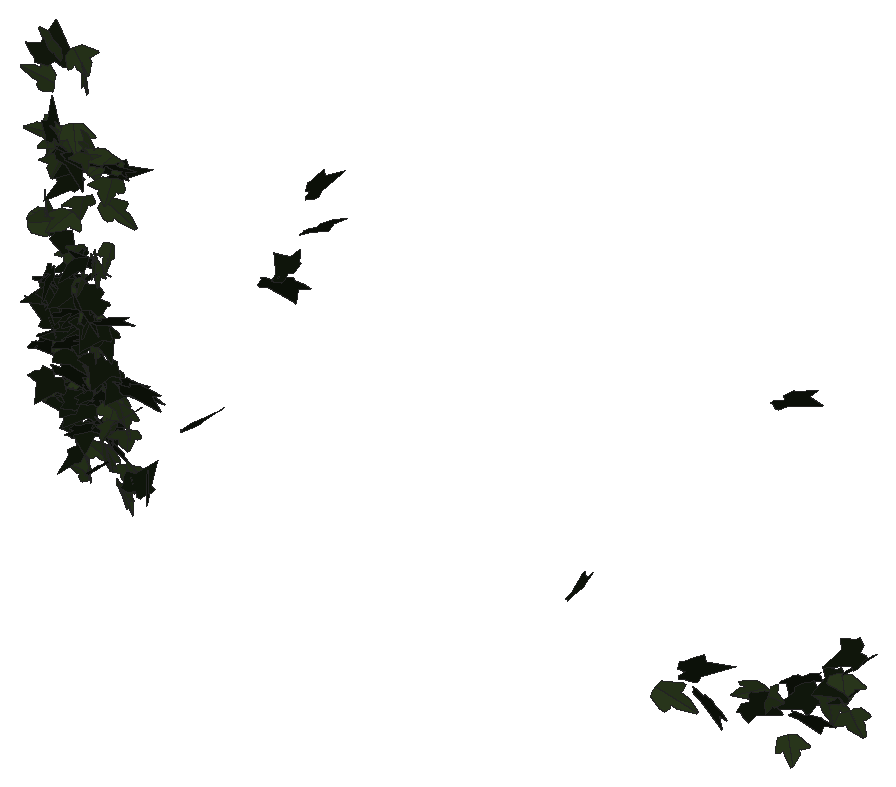
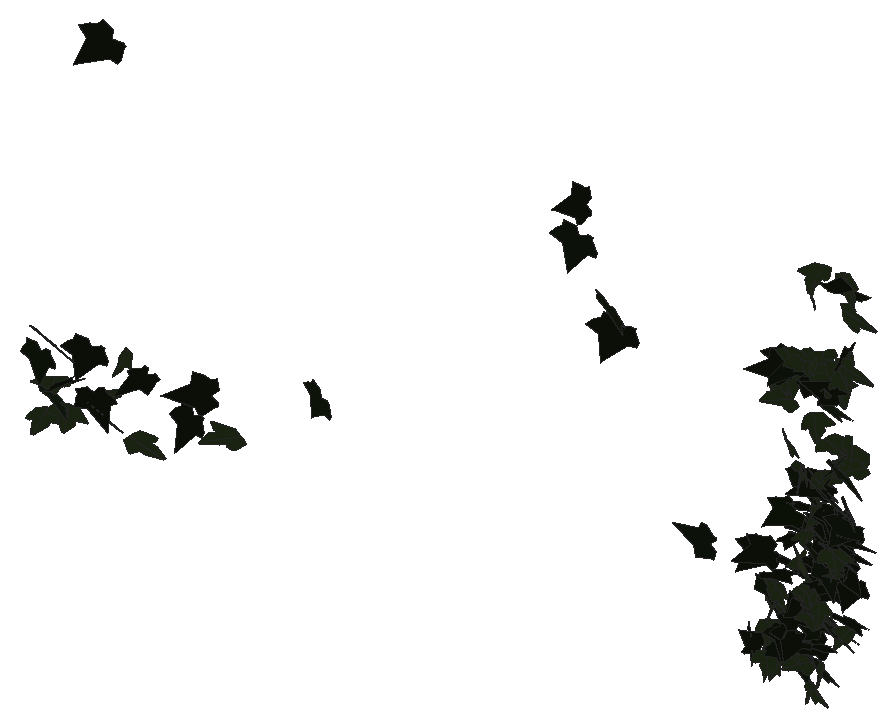
# SketchUp Ruby script. Lengths in inches.
U = 1.inch
M = Sketchup.active_model
def pt(a) = Geom::Point3d.new(a.map { |v| v * U })
def face(e, loops, mat)
  f = e.add_face(loops[0].map { |a| pt(a) })
  loops[1..].each { |l| e.add_face(l.map { |a| pt(a) }).erase! }
  f.material = f.back_material = mat if mat
  f
end
# faces: each face lists its corners as indices into pts; further lists are holes
def faces(e, pts, list, mat = nil) = list.each { |f| face(e, (f[0].is_a?(Array) ? f : [f]).map { |l| l.map { |i| pts[i] } }, mat) }
# xy, xz, yz: faces in a plane at the given z, y or x. An outline is a flat list of corners, or four numbers for a rectangle; further outlines are holes
def ring(l) = l.size == 4 ? [[l[0], l[1]], [l[2], l[1]], [l[2], l[3]], [l[0], l[3]]] : l.each_slice(2).to_a
def flat(e, list, mat, &to3) = list.each { |f| face(e, (f[0].is_a?(Array) ? f : [f]).map { |l| ring(l).map { |u, v| to3.(u, v) } }, mat) }
def xy(e, z, list, mat = nil) = flat(e, list, mat) { |x, y| [x, y, z] }
def xz(e, y, list, mat = nil) = flat(e, list, mat) { |x, z| [x, y, z] }
def yz(e, x, list, mat = nil) = flat(e, list, mat) { |y, z| [x, y, z] }
def lines(e, pts, list) = list.each { |a, b| e.add_line(pt(pts[a]), pt(pts[b])) }
# prism: a flat outline (further loops are holes) pulled along v
def prism(e, loops, v, mat = nil)
  f = face(e, loops, mat); d = Geom::Vector3d.new(v.map { |x| x * U })
  f.pushpull(f.normal.samedirection?(d) ? d.length : -d.length)
end
def box(e, o, s, mat = nil) = prism(e, [[o, [o[0] + s[0], o[1], o[2]], [o[0] + s[0], o[1] + s[1], o[2]], [o[0], o[1] + s[1], o[2]]]], [0, 0, s[2]], mat)
def at(x, y, z, deg = 0) = Geom::Transformation.translation(pt([x, y, z])) * Geom::Transformation.rotation(ORIGIN, Z_AXIS, deg.degrees)
def axes(o, x, y, z) = Geom::Transformation.new([*x, 0, *y, 0, *z, 0, *pt(o).to_a, 1])
def part(name) = M.definitions.add(name)
# library, detail: a bought-in or finely detailed component or shape, given as its bounding box
def library(name, o, s) = part(name).tap { |d| box(d.entities, o, s) }
def detail(e, o, s) = box(e.add_group.entities, o, s)
def put(e, d, t, mat = nil) = e.add_instance(d, t).tap { |i| i.material = mat if mat }
def group(e, t, mat = nil) = e.add_group.tap { |g| g.transformation = t; g.material = mat if mat }.entities
root = M.entities
M.materials.add("1026 AP 7946 SUNNY SIDE UP").color = [254, 231, 186]
M.materials.add("efeu1").color = [18, 25, 13]
M.materials.add("efeu2").color = [43, 57, 29]
c1 = part("ivyleaf_10")
p = [[0,0.5,-0.03],[-0.0625,2.02,-0.43],[-0.19,2.01,-0.46],[-0.54,1.05,-0.29],[-0.52,0.625,-0.18],[-0.83,0.76,-0.28],
  [-1.16,0.64,-0.33],[-1.15,0.33,-0.24],[-0.77,-0.39,0.02],[-0.3,-0.51,0.16],[0.04,-0.48,0.23],[-0.02,2.01,-0.4375],
  [-0.06,2.01,-0.43],[0.04,-0.49,0.23],[0.67,-0.49,0.14],[1.38,0.36,-0.2],[1.375,0.51,-0.24],[0.81,0.65,-0.19],
  [0.62,0.59,-0.15],[0.6,1.09,-0.28],[0.5,1.23,-0.31]]
faces(c1.entities,p,[[0,1,2,3,4,5,6,7,8,9,10],[11,12,0,13,14,15,16,17,18,19,20]],"efeu2")
c2 = part("ivyleaf_9")
p = [[1.54,2.16,1.25],[1.36,2.04,1.19],[-0.21,0.99,0.68],[-0.71,1.11,0.82],[-0.85,0.86,0.67],[-0.8,0.17,0.21],
  [-0.9,-0.01,0.1],[-0.67,-0.16,-0.02],[-0.08,-0.08,-0.05],[-0.03,-0.6,-0.4],[0.65,-0.88,-0.66],[0.83,-0.6,-0.49],
  [1.29,-0.42,-0.43],[1.8125,-0.07,-0.26],[1.21,0.44,0.15]]
faces(c2.entities,p,[[0,1,2,3,4,5,6,7,8,9,10,11,12,13,14]],"efeu1")
put(root,c1,axes([98.42,213.14,277.24],[0.01091,0.05162,0.27942],[-0.44913,0.02167,0.0027],[-0.03534,-0.2595,0.05202]),"1026 AP 7946 SUNNY SIDE UP")
put(root,c1,axes([98.55,213.2,275.9],[-0.07101,0.03292,0.2675],[-0.42315,-0.03971,-0.0397],[0.05791,-0.24978,0.03794]),"1026 AP 7946 SUNNY SIDE UP")
put(root,c1,axes([98.3125,213.24,274.14],[-0.23454,0.18097,0.09974],[-0.13964,0.05028,-0.24058],[-0.31407,-0.1575,0.03248]),"1026 AP 7946 SUNNY SIDE UP")
put(root,c1,axes([98.02,213.31,273.63],[0.17305,0.09582,0.20323],[0.2394,0.12524,-0.14799],[-0.26763,0.17399,-0.00097]),"1026 AP 7946 SUNNY SIDE UP")
put(root,c1,axes([98.4375,213.24,278.14],[-0.33536,0.12077,0.14156],[-0.23164,0.02245,-0.24278],[-0.19382,-0.23579,0.04521]),"1026 AP 7946 SUNNY SIDE UP")
put(root,c2,axes([98.49,213.48,271.78],[-0.34588,-0.02797,0.10109],[-0.14748,-0.05284,-0.21736],[0.07996,-0.21842,0.03636]),"1026 AP 7946 SUNNY SIDE UP")
put(root,c2,axes([98.21,213.35,272.16],[0.28691,0.14385,0.05154],[0.01081,0.06257,-0.23231],[-0.25628,0.16368,0.0479]),"1026 AP 7946 SUNNY SIDE UP")
put(root,c2,axes([98.27,213.1875,270.64],[0.2103,0.18763,-0.0042],[0.01051,-0.01171,-0.24055],[-0.31852,0.12349,-0.01071]),"1026 AP 7946 SUNNY SIDE UP")
put(root,c2,axes([98.5,213.48,273.58],[-0.24446,0.18597,-0.01038],[-0.00582,-0.01796,-0.25164],[-0.31631,-0.1434,0.01265]),"1026 AP 7946 SUNNY SIDE UP")
put(root,c1,axes([98.17,213.02,273.62],[-0.00352,-0.01577,0.26143],[0.1187,0.23419,0.02008],[-0.39843,0.06991,0.00367]),"1026 AP 7946 SUNNY SIDE UP")
put(root,c2,axes([98.65,213.15,271.35],[-0.11475,0.11007,0.21516],[-0.25252,0.13636,-0.13257],[-0.29305,-0.1606,0.02999]),"1026 AP 7946 SUNNY SIDE UP")
put(root,c2,axes([98.44,213.28,269.74],[-0.33804,-0.05996,-0.05433],[0.09397,-0.01196,-0.22097],[0.09341,-0.20496,0.02568]),"1026 AP 7946 SUNNY SIDE UP")
put(root,c1,axes([98.34,213.3,269.43],[0.08571,0.15443,0.15045],[-0.00221,0.14279,-0.16793],[-0.35215,0.03669,0.03767]),"1026 AP 7946 SUNNY SIDE UP")
put(root,c2,axes([98.4375,213.1,271.4],[0.20472,-0.0542,-0.20479],[-0.29694,0.07567,-0.14048],[0.15798,0.21246,0.00133]),"1026 AP 7946 SUNNY SIDE UP")
put(root,c1,axes([98.49,213.35,275.81],[0.03464,0.23008,-0.09791],[-0.14517,-0.0825,-0.23609],[-0.39646,0.05031,0.07789]),"1026 AP 7946 SUNNY SIDE UP")
put(root,c2,axes([98.6,213.23,270.97],[-0.01316,0.1754,-0.14964],[-0.05252,-0.14163,-0.18737],[-0.37954,0.01352,0.03112]),"1026 AP 7946 SUNNY SIDE UP")
put(root,c2,axes([98.55,213.21,277.77],[-0.42037,0.02729,0.08947],[0.14494,0.01969,0.26537],[0.03308,0.2605,-0.02574]),"1026 AP 7946 SUNNY SIDE UP")
put(root,c2,axes([98.42,213.22,272.4375],[-0.20286,0.03865,-0.21315],[0.29531,-0.10039,-0.13371],[-0.17862,-0.20987,0.02101]),"1026 AP 7946 SUNNY SIDE UP")
put(root,c1,axes([98.61,213.22,275.73],[-0.21138,-0.17852,-0.14178],[-0.15191,-0.09578,0.23105],[-0.34284,0.15251,-0.01497]),"1026 AP 7946 SUNNY SIDE UP")
put(root,c2,axes([98.51,213.375,272.24],[0.27432,0.15021,-0.04954],[-0.03663,-0.04736,-0.23593],[-0.26529,0.16186,-0.01865]),"1026 AP 7946 SUNNY SIDE UP")
put(root,c2,axes([98.48,213.49,271.73],[-0.18652,-0.19675,0.02288],[0.06417,-0.04767,-0.23437],[0.33028,-0.10185,0.05846]),"1026 AP 7946 SUNNY SIDE UP")
put(root,c1,axes([98.6,213.47,271.35],[-0.2889,-0.1418,0.03043],[-0.00796,-0.04127,-0.23577],[0.24601,-0.16786,0.02811]),"1026 AP 7946 SUNNY SIDE UP")
put(root,c2,axes([98.72,213.48,269.5625],[-0.27699,0.12648,-0.04289],[0.03306,-0.04259,-0.22043],[-0.22364,-0.16294,0.02053]),"1026 AP 7946 SUNNY SIDE UP")
put(root,c2,axes([98.58,213.34,272.32],[0.17219,0.19894,-0.03572],[-0.01358,-0.03625,-0.23937],[-0.34291,0.10133,-0.00846]),"1026 AP 7946 SUNNY SIDE UP")
put(root,c2,axes([98.63,213.08,275.96],[-0.12376,-0.12351,0.23299],[0.1538,0.20006,0.15571],[-0.39851,0.11557,-0.01226]),"1026 AP 7946 SUNNY SIDE UP")
put(root,c1,axes([98.59,213.48,270.85],[0.18494,0.14833,-0.13167],[-0.10181,-0.11049,-0.198],[-0.31307,0.12356,-0.0134]),"1026 AP 7946 SUNNY SIDE UP")
put(root,c2,axes([98.9,213.25,271.31],[-0.15454,0.17398,0.12199],[-0.18019,0.06538,-0.20077],[-0.30117,-0.12839,0.05752]),"1026 AP 7946 SUNNY SIDE UP")
put(root,c2,axes([98.75,213.51,270.94],[-0.00684,0.22013,-0.00663],[0.00213,-0.00904,-0.23582],[-0.37398,-0.00408,-0.00122]),"1026 AP 7946 SUNNY SIDE UP")
put(root,c1,axes([98.75,213.17,275.4],[-0.18203,-0.22494,0.06303],[-0.02963,-0.0601,-0.26742],[0.39489,-0.1082,0.00899]),"1026 AP 7946 SUNNY SIDE UP")
put(root,c2,axes([98.82,213.28,273.22],[-0.13782,-0.18844,0.13747],[0.0698,0.12462,0.22116],[-0.38315,0.09049,-0.00916]),"1026 AP 7946 SUNNY SIDE UP")
put(root,c1,axes([98.88,213.23,273.96],[0.2441,0.12071,-0.15989],[-0.21585,-0.08257,-0.20155],[-0.24705,0.19141,0.01812]),"1026 AP 7946 SUNNY SIDE UP")
put(root,c2,axes([99.11,213.12,269.4],[-0.23979,0.13123,0.11003],[-0.16609,0.04107,-0.20292],[-0.22688,-0.16877,0.03226]),"1026 AP 7946 SUNNY SIDE UP")
put(root,c1,axes([98.86,213.53,268.44],[-0.1644,0.1814,0.02826],[-0.03976,0.01468,-0.21946],[-0.30807,-0.0987,0.01324]),"1026 AP 7946 SUNNY SIDE UP")
put(root,c2,axes([98.68,213.23,275.1875],[0.00522,0.01474,0.26959],[0.38782,0.10615,-0.00817],[-0.18076,0.22816,-0.00974]),"1026 AP 7946 SUNNY SIDE UP")
put(root,c2,axes([99.1,213.37,271.33],[-0.18583,0.1867,-0.06559],[-0.0432,-0.08561,-0.223],[-0.33207,-0.09334,0.06571]),"1026 AP 7946 SUNNY SIDE UP")
put(root,c1,axes([98.82,213.41,270.95],[-0.25607,0.1361,-0.08408],[0.08371,-0.06494,-0.21789],[-0.25486,-0.15808,0.0129]),"1026 AP 7946 SUNNY SIDE UP")
put(root,c1,axes([98.92,213.54,269.96],[-0.08133,-0.19713,-0.07825],[0.03355,0.06776,-0.21622],[0.35382,-0.05174,0.00252]),"1026 AP 7946 SUNNY SIDE UP")
put(root,c2,axes([99.03,213.29,274.92],[-0.37212,0.0347,-0.1109],[0.12555,-0.12493,-0.21318],[-0.13748,-0.20802,0.1055]),"1026 AP 7946 SUNNY SIDE UP")
put(root,c1,axes([99.18,213.36,275.6],[-0.26887,-0.00386,-0.20285],[-0.32043,-0.01799,0.16912],[-0.02763,0.24626,0.01263]),"1026 AP 7946 SUNNY SIDE UP")
put(root,c2,axes([99.12,213.41,272.88],[-0.31302,0.14344,-0.02423],[0.00867,-0.03315,-0.24937],[-0.24688,-0.18304,0.02196]),"1026 AP 7946 SUNNY SIDE UP")
put(root,c1,axes([98.96,213.36,273.1],[-0.17934,-0.21396,0.00359],[0.02548,-0.01424,-0.25479],[0.36246,-0.10486,0.01969]),"1026 AP 7946 SUNNY SIDE UP")
put(root,c2,axes([99.1,213.36,272.13],[-0.34503,-0.09445,0.06474],[-0.07489,-0.05048,-0.239],[0.17627,-0.20633,0.02518]),"1026 AP 7946 SUNNY SIDE UP")
put(root,c2,axes([98.85,213.13,271.6],[0.23886,0.16278,0.08406],[0.11432,0.04224,-0.22856],[-0.28304,0.15444,-0.02137]),"1026 AP 7946 SUNNY SIDE UP")
put(root,c2,axes([99.2,213.375,271.03],[-0.05721,-0.07875,-0.22458],[-0.17181,-0.18275,0.08875],[-0.33753,0.10637,-0.00711]),"1026 AP 7946 SUNNY SIDE UP")
put(root,c2,axes([98.88,213.42,270.48],[-0.13472,-0.16506,-0.12476],[0.14192,0.08467,-0.19172],[0.30994,-0.11051,0.03356]),"1026 AP 7946 SUNNY SIDE UP")
put(root,c1,axes([99.27,213.34,267.71],[-0.03561,0.06083,0.21514],[-0.33094,0.06729,-0.04282],[-0.12882,-0.18968,0.05055]),"1026 AP 7946 SUNNY SIDE UP")
put(root,c2,axes([98.87,213.3,275.42],[0.05181,-0.23965,0.06411],[0.06263,-0.05838,-0.25767],[0.41595,0.03864,0.03081]),"1026 AP 7946 SUNNY SIDE UP")
put(root,c2,axes([99.03,212.98,271.01],[0.18245,0.19127,0.05617],[0.06019,0.03731,-0.23399],[-0.33014,0.11251,-0.01161]),"1026 AP 7946 SUNNY SIDE UP")
put(root,c1,axes([99.05,213.35,272.18],[-0.00436,0.12431,0.21121],[-0.05002,0.19392,-0.1296],[-0.39033,-0.02624,0.01425]),"1026 AP 7946 SUNNY SIDE UP")
put(root,c1,axes([99.01,213.3,276.11],[0.22437,0.21306,-0.01588],[0.00324,-0.02188,-0.26837],[-0.36291,0.13153,-0.01221]),"1026 AP 7946 SUNNY SIDE UP")
put(root,c2,axes([99.33,213.06,269.55],[-0.06414,0.1623,0.14715],[-0.19669,0.09906,-0.16043],[-0.3,-0.09965,0.07373]),"1026 AP 7946 SUNNY SIDE UP")
put(root,c2,axes([98.93,213.03,270.27],[0.3751,0.04298,0.01044],[0.02254,-0.02038,-0.24007],[-0.07113,0.22022,-0.02103]),"1026 AP 7946 SUNNY SIDE UP")
put(root,c2,axes([99.1875,213.32,273],[-0.33758,0.06627,-0.11299],[0.15423,-0.0613,-0.2235],[-0.14662,-0.21706,0.02506]),"1026 AP 7946 SUNNY SIDE UP")
put(root,c2,axes([99.23,213.37,275.48],[-0.01147,0.0781,-0.25158],[-0.00822,-0.23609,-0.08679],[-0.42193,0.00248,0.00853]),"1026 AP 7946 SUNNY SIDE UP")
put(root,c2,axes([99.28,213.4,269.79],[-0.24975,0.15103,-0.04751],[0.01152,-0.05723,-0.22353],[-0.26794,-0.14324,0.03467]),"1026 AP 7946 SUNNY SIDE UP")
put(root,c1,axes([99.08,213.51,269.62],[0.32783,0.09105,-0.02043],[-0.03132,-0.00841,-0.2287],[-0.15522,0.194,0.00299]),"1026 AP 7946 SUNNY SIDE UP")
put(root,c2,axes([99.36,213.41,269.75],[-0.24506,0.16486,0.02906],[-0.05668,0.00381,-0.23331],[-0.27731,-0.14646,0.022]),"1026 AP 7946 SUNNY SIDE UP")
put(root,c2,axes([99.29,213.33,271.72],[-0.33296,0.0957,-0.06859],[0.08617,-0.04447,-0.23356],[-0.17681,-0.2019,0.01534]),"1026 AP 7946 SUNNY SIDE UP")
put(root,c2,axes([98.9,213.35,272.93],[0.3752,0.01236,0.08152],[0.12805,0.01142,-0.23673],[-0.02613,0.23345,0.01054]),"1026 AP 7946 SUNNY SIDE UP")
put(root,c2,axes([99.26,213.18,268.25],[-0.2801,0.07554,-0.11272],[0.129,-0.08357,-0.19108],[-0.17986,-0.17758,0.03849]),"1026 AP 7946 SUNNY SIDE UP")
put(root,c1,axes([99.22,213.32,274.44],[-0.19893,-0.21213,-0.00644],[0.02394,-0.00409,-0.25906],[0.35935,-0.11716,0.01369]),"1026 AP 7946 SUNNY SIDE UP")
put(root,c2,axes([99.27,213.32,269.38],[-0.31837,-0.11313,0.00521],[0.00769,-0.01974,-0.23386],[0.19219,-0.18662,0.01799]),"1026 AP 7946 SUNNY SIDE UP")
put(root,c1,axes([99.18,213.55,267.82],[-0.15731,0.1739,-0.04406],[0.0011,-0.04856,-0.21035],[-0.30427,-0.09009,0.02202]),"1026 AP 7946 SUNNY SIDE UP")
put(root,c2,axes([98.97,213.48,269.32],[0.135,-0.15384,0.12693],[0.14886,-0.08825,-0.18371],[0.29653,0.11434,0.03444]),"1026 AP 7946 SUNNY SIDE UP")
put(root,c1,axes([99.24,213.27,272.5],[0.06503,-0.16046,-0.18531],[0.01886,0.17432,-0.17002],[0.39763,0.01797,0.03837]),"1026 AP 7946 SUNNY SIDE UP")
put(root,c1,axes([99.18,213.19,278.11],[0.17467,0.22446,0.11823],[-0.00278,0.11694,-0.25808],[-0.42247,0.09203,0.05058]),"1026 AP 7946 SUNNY SIDE UP")
put(root,c2,axes([99.1875,213.37,268.85],[-0.19728,-0.15667,-0.08755],[0.13412,0.03884,-0.20444],[0.26658,-0.13548,0.03806]),"1026 AP 7946 SUNNY SIDE UP")
put(root,c1,axes([99.22,213.4,275.99],[-0.25345,0.18525,-0.08341],[0.06253,-0.07323,-0.25514],[-0.337,-0.15291,0.01539]),"1026 AP 7946 SUNNY SIDE UP")
put(root,c1,axes([99.27,213.4,270.16],[-0.26898,0.14677,-0.05577],[0.05243,-0.04601,-0.23149],[-0.26025,-0.16096,0.01101]),"1026 AP 7946 SUNNY SIDE UP")
put(root,c2,axes([99.17,213.13,268.76],[0.21139,0.09661,0.15308],[0.19214,0.08532,-0.16754],[-0.21879,0.16828,0.00078]),"1026 AP 7946 SUNNY SIDE UP")
put(root,c1,axes([99.16,213.44,277.57],[0.05577,-0.07832,0.2568],[0.29269,-0.17104,-0.08709],[0.31501,0.17279,0.03546]),"1026 AP 7946 SUNNY SIDE UP")
put(root,c2,axes([99.61,213.16,269.84],[-0.16784,0.18845,0.0398],[-0.08932,0.01087,-0.22341],[-0.31278,-0.10423,0.04244]),"1026 AP 7946 SUNNY SIDE UP")
put(root,c1,axes([99.34,213.4,271.61],[0.11657,0.21521,-0.02247],[-0.0107,-0.02296,-0.24216],[-0.3674,0.06895,-0.00008]),"1026 AP 7946 SUNNY SIDE UP")
put(root,c1,axes([99.4375,213.48,270.04],[-0.2926,0.13445,0.00155],[-0.03607,-0.02773,-0.23141],[-0.22537,-0.17012,0.03503]),"1026 AP 7946 SUNNY SIDE UP")
put(root,c2,axes([99.66,213.32,272.15],[-0.37347,-0.01953,0.08498],[-0.12339,-0.05902,-0.23133],[0.06439,-0.22641,0.04958]),"1026 AP 7946 SUNNY SIDE UP")
put(root,c2,axes([99.26,213.28,271.93],[0.13314,-0.21709,0.03927],[0.01668,-0.03846,-0.24762],[0.3742,0.07896,-0.00294]),"1026 AP 7946 SUNNY SIDE UP")
put(root,c1,axes([99.23,213.37,270.22],[0.1824,-0.04857,0.20502],[0.29323,-0.08417,-0.12737],[0.16488,0.20341,-0.00027]),"1026 AP 7946 SUNNY SIDE UP")
put(root,c2,axes([99.71,213.29,271.35],[-0.35847,0.06724,0.04138],[-0.08211,-0.0297,-0.23329],[-0.10197,-0.21245,0.04239]),"1026 AP 7946 SUNNY SIDE UP")
put(root,c2,axes([99.53,213.48,269.59],[-0.18808,-0.0704,0.18115],[0.21615,0.11411,0.14093],[-0.22574,0.16791,-0.01599]),"1026 AP 7946 SUNNY SIDE UP")
put(root,c1,axes([99.42,213.48,270.75],[0.17882,-0.18855,-0.05745],[0.06185,-0.03819,0.23028],[-0.32585,-0.11072,0.01218]),"1026 AP 7946 SUNNY SIDE UP")
put(root,c2,axes([99.73,213.27,272.88],[-0.16545,0.21672,-0.03522],[0.00704,-0.03726,-0.25463],[-0.3728,-0.09689,0.01082]),"1026 AP 7946 SUNNY SIDE UP")
put(root,c1,axes([99.57,213.32,273.02],[0.09673,-0.17129,-0.17431],[0.02752,0.16772,-0.18303],[0.39762,0.03006,0.05507]),"1026 AP 7946 SUNNY SIDE UP")
put(root,c1,axes([99.6,213.1875,275.66],[-0.40177,-0.09274,-0.01618],[0.03577,-0.01581,-0.27131],[0.15512,-0.23656,0.02066]),"1026 AP 7946 SUNNY SIDE UP")
put(root,c1,axes([99.55,213.45,270.9375],[0.05493,0.20859,-0.0695],[-0.01153,-0.06738,-0.2269],[-0.37206,0.03288,-0.00323]),"1026 AP 7946 SUNNY SIDE UP")
put(root,c2,axes([99.51,213.52,269.37],[0.23617,0.129,0.10588],[-0.15484,-0.04315,0.20044],[0.2263,-0.16415,0.02665]),"1026 AP 7946 SUNNY SIDE UP")
put(root,c1,axes([99.62,213.29,273.01],[-0.29515,0.16628,-0.02064],[-0.03681,-0.05293,-0.25196],[-0.28221,-0.167,0.05445]),"1026 AP 7946 SUNNY SIDE UP")
put(root,c2,axes([99.68,213.25,271.51],[-0.32744,-0.11249,-0.0349],[0.09405,-0.03532,-0.23138],[0.17439,-0.19217,0.05926]),"1026 AP 7946 SUNNY SIDE UP")
put(root,c1,axes([99.4375,213.4,268.34],[0.21584,0.0178,0.17543],[0.23762,0.09709,-0.12639],[-0.14701,0.18307,0.05327]),"1026 AP 7946 SUNNY SIDE UP")
put(root,c2,axes([99.62,213.49,269.02],[0.27905,0.12389,-0.04865],[-0.03842,-0.04763,-0.21956],[-0.22167,0.16422,-0.02319]),"1026 AP 7946 SUNNY SIDE UP")
put(root,c2,axes([99.7,213.35,271.41],[-0.04935,-0.21517,-0.09109],[0.02653,0.0809,-0.23127],[0.39015,-0.03272,0.0042]),"1026 AP 7946 SUNNY SIDE UP")
put(root,c1,axes([100.01,213.26,275.76],[-0.3453,-0.04576,0.15662],[-0.1786,-0.13631,-0.20333],[0.19057,-0.21065,0.09324]),"1026 AP 7946 SUNNY SIDE UP")
put(root,c2,axes([99.95,213.03,268.22],[-0.04827,0.20732,-0.03934],[-0.00363,-0.04009,-0.22445],[-0.35823,-0.02753,0.00757]),"1026 AP 7946 SUNNY SIDE UP")
put(root,c2,axes([99.86,213.29,270.66],[-0.33052,-0.09159,-0.075],[0.1211,0.00935,-0.22914],[0.15222,-0.20631,0.01946]),"1026 AP 7946 SUNNY SIDE UP")
put(root,c1,axes([99.89,213.36,268.45],[-0.31638,0.08926,0.01553],[-0.04075,-0.01952,-0.21948],[-0.14768,-0.18583,0.02729]),"1026 AP 7946 SUNNY SIDE UP")
put(root,c2,axes([99.875,213.41,268.93],[0.26871,0.13141,-0.06987],[-0.06106,-0.06089,-0.21976],[-0.24282,0.16073,-0.02206]),"1026 AP 7946 SUNNY SIDE UP")
put(root,c1,axes([99.89,213.4,269.1],[-0.11069,0.20301,-0.0359],[0.00156,-0.03766,-0.22852],[-0.35004,-0.06436,0.01033]),"1026 AP 7946 SUNNY SIDE UP")
put(root,c1,axes([100.06,213.27,275.17],[-0.24975,-0.19503,0.06288],[0.01592,-0.08186,-0.25595],[0.34666,-0.13675,0.05706]),"1026 AP 7946 SUNNY SIDE UP")
put(root,c1,axes([99.95,213.41,269.42],[0.35294,-0.05996,0.03282],[0.04009,-0.03094,-0.23078],[0.10771,0.20799,-0.02166]),"1026 AP 7946 SUNNY SIDE UP")
put(root,c1,axes([100.1,213.15,268.51],[-0.23174,0.15788,0.05129],[-0.06964,0.025,-0.22257],[-0.27026,-0.14182,0.01337]),"1026 AP 7946 SUNNY SIDE UP")
put(root,c2,axes([99.96,213.16,275.6],[0.3649,0.13413,0.01626],[-0.0139,0.03824,-0.26786],[-0.22841,0.21196,0.04228]),"1026 AP 7946 SUNNY SIDE UP")
put(root,c1,axes([100.14,213.18,269.24],[-0.05388,-0.19465,0.0931],[-0.00476,-0.09009,-0.21208],[0.36365,-0.03002,0.01102]),"1026 AP 7946 SUNNY SIDE UP")
put(root,c2,axes([99.98,213.12,271.79],[0.29245,0.11477,0.11414],[0.10679,0.09207,-0.21672],[-0.24165,0.17959,0.04236]),"1026 AP 7946 SUNNY SIDE UP")
put(root,c1,axes([100.05,213.2,273.55],[0.27474,-0.15106,0.10368],[0.11089,-0.07471,-0.23785],[0.28564,0.17429,-0.00739]),"1026 AP 7946 SUNNY SIDE UP")
put(root,c2,axes([100,213.4375,268.55],[0.29931,-0.11568,0.03028],[0.02024,-0.03581,-0.2249],[0.20177,0.1752,-0.02236]),"1026 AP 7946 SUNNY SIDE UP")
put(root,c2,axes([100.3,213.41,270.28],[-0.26281,-0.15665,0.0324],[-0.02537,-0.0306,-0.23593],[0.27033,-0.15516,0.00936]),"1026 AP 7946 SUNNY SIDE UP")
put(root,c2,axes([100.07,213.3,275.39],[0.15261,0.0879,0.23489],[0.32062,0.11237,-0.13018],[-0.23819,0.20758,-0.02473]),"1026 AP 7946 SUNNY SIDE UP")
put(root,c1,axes([100.375,213.43,268.98],[-0.24164,-0.16003,-0.01606],[0.04041,-0.00397,-0.2283],[0.26952,-0.14287,0.01983]),"1026 AP 7946 SUNNY SIDE UP")
put(root,c1,axes([100.06,213.24,274.62],[0.2185,0.02688,0.22589],[0.34509,0.05561,-0.13981],[-0.10421,0.24051,0.01066]),"1026 AP 7946 SUNNY SIDE UP")
put(root,c1,axes([100.33,213.41,269.39],[-0.10757,0.20262,-0.04918],[0.02219,-0.04681,-0.22793],[-0.35301,-0.06469,0.00066]),"1026 AP 7946 SUNNY SIDE UP")
put(root,c1,axes([100.46,213.41,268.15],[-0.27905,-0.12921,-0.00718],[0.02522,-0.01081,-0.22319],[0.21805,-0.1641,0.01663]),"1026 AP 7946 SUNNY SIDE UP")
put(root,c1,axes([100.27,213.36,269.81],[0.25545,-0.09512,0.13753],[0.22274,-0.03013,-0.18706],[0.15792,0.19637,0.04136]),"1026 AP 7946 SUNNY SIDE UP")
put(root,c1,axes([100.49,213.14,269.78],[-0.36124,0.05342,-0.00566],[0.00095,-0.02222,-0.23408],[-0.09125,-0.21172,0.01996]),"1026 AP 7946 SUNNY SIDE UP")
put(root,c1,axes([100.52,213.09,267.85],[-0.28659,0.14699,-0.01067],[-0.0057,-0.02188,-0.23911],[-0.25026,-0.16782,0.01766]),"1026 AP 7946 SUNNY SIDE UP")
put(root,c2,axes([100.71,213.04,269.72],[-0.03286,0.23232,0.00526],[-0.01035,0.00138,-0.24948],[-0.39425,-0.0194,0.00611]),"1026 AP 7946 SUNNY SIDE UP")
put(root,c1,axes([100.64,213.08,267.74],[-0.08595,0.21408,0.01167],[-0.00328,0.00787,-0.2354],[-0.36366,-0.05067,-0.00064]),"1026 AP 7946 SUNNY SIDE UP")
put(root,c1,axes([100.72,213.07,268.34],[-0.14547,0.20636,-0.01209],[-0.00259,-0.01576,-0.2393],[-0.3511,-0.08538,0.00678]),"1026 AP 7946 SUNNY SIDE UP")
put(root,c2,axes([100.67,213.01,270.51],[0.37832,0.02359,0.08587],[0.13544,0.00528,-0.23983],[-0.04072,0.2367,0.00013]),"1026 AP 7946 SUNNY SIDE UP")
put(root,c2,axes([100.86,213,270.47],[0.38954,0.07582,0.01506],[0.03422,-0.01953,-0.25763],[-0.12604,0.22901,-0.02339]),"1026 AP 7946 SUNNY SIDE UP")
put(root,c2,axes([101.01,212.96,268.04],[-0.11778,-0.03216,0.25213],[0.30501,0.15081,0.0824],[-0.24051,0.20701,-0.01897]),"1026 AP 7946 SUNNY SIDE UP")
put(root,c2,axes([101.33,212.95,268.29],[0.05475,-0.01803,-0.26459],[-0.36345,0.11174,-0.03973],[0.17797,0.23375,0.00027]),"1026 AP 7946 SUNNY SIDE UP")
put(root,c2,axes([102.44,212.97,270.07],[0.0534,0.25988,-0.05212],[0.01382,0.05136,0.2703],[0.41653,-0.03502,-0.00228]),"1026 AP 7946 SUNNY SIDE UP")
put(root,c2,axes([104.91,212.98,274.56],[0.35207,0.17698,-0.03229],[-0.02099,-0.03515,-0.29356],[-0.28211,0.22348,-0.01845]),"1026 AP 7946 SUNNY SIDE UP")
put(root,c2,axes([105.25,212.92,274.95],[-0.05841,0.21133,0.20502],[-0.11115,0.18678,-0.21814],[-0.44137,-0.075,0.02781]),"1026 AP 7946 SUNNY SIDE UP")
put(root,c2,axes([105.93,212.91,277.24],[0.08653,0.10076,0.28718],[0.26926,0.21991,-0.11566],[-0.37939,0.17905,-0.01659]),"1026 AP 7946 SUNNY SIDE UP")
put(root,c2,axes([106.1,212.91,276.38],[0.17218,0.26862,0.07243],[0.01247,0.07089,-0.29779],[-0.43582,0.10815,0.02009]),"1026 AP 7946 SUNNY SIDE UP")
put(root,c2,axes([113.28,212.88,269.83],[0.06734,0.16983,0.23206],[0.02536,0.22502,-0.17738],[-0.44164,0.03882,0.0252]),"1026 AP 7946 SUNNY SIDE UP")
put(root,c1,axes([115.63,213.01,268.09],[0.16562,0.10642,0.26383],[0.32092,0.15478,-0.15219],[-0.29394,0.22894,-0.0175]),"1026 AP 7946 SUNNY SIDE UP")
put(root,c2,axes([116.3,212.98,268.88],[0.19438,0.08894,0.26631],[0.35282,0.12809,-0.1555],[-0.24424,0.25581,-0.01268]),"1026 AP 7946 SUNNY SIDE UP")
put(root,c2,axes([116.66,213.12,268.27],[0.41484,-0.04348,-0.14328],[-0.22036,0.00128,-0.27474],[0.06145,0.29812,-0.01794]),"1026 AP 7946 SUNNY SIDE UP")
put(root,c1,axes([117.16,214.41,268.09],[0.21546,0.07797,-0.20843],[-0.33094,-0.01172,-0.15124],[-0.08459,0.24444,0.06081]),"1026 AP 7946 SUNNY SIDE UP")
put(root,c2,axes([118.09,212.95,268.74],[0.04504,-0.0156,-0.26719],[-0.06931,0.25677,-0.01943],[0.40249,0.04596,0.02655]),"1026 AP 7946 SUNNY SIDE UP")
put(root,c2,axes([118.34,214.41,268.81],[0.05169,0.23186,-0.11308],[-0.04224,-0.10828,-0.24165],[-0.40205,0.04119,0.01085]),"1026 AP 7946 SUNNY SIDE UP")
put(root,c2,axes([118.64,214.34,268.47],[-0.38801,0.09537,0.0219],[-0.04406,-0.01529,-0.27148],[-0.14699,-0.24716,0.02358]),"1026 AP 7946 SUNNY SIDE UP")
put(root,c1,axes([118.625,212.97,269.05],[0.01317,-0.16936,-0.20722],[0.09867,0.19576,-0.16677],[0.40034,-0.04268,0.04792]),"1026 AP 7946 SUNNY SIDE UP")
put(root,c1,axes([118.92,214.63,268.32],[-0.40047,-0.04337,-0.01194],[0.02553,-0.02825,-0.26445],[0.06571,-0.25337,0.02999]),"1026 AP 7946 SUNNY SIDE UP")
put(root,c1,axes([119.02,213.11,268.01],[0.20453,0.22182,-0.00296],[0.01449,-0.01019,-0.26462],[-0.34855,0.12974,-0.01274]),"1026 AP 7946 SUNNY SIDE UP")
put(root,c2,axes([119.33,214.64,268.58],[-0.03783,0.21351,0.15237],[-0.13777,0.13193,-0.21186],[-0.38332,-0.06849,0.06111]),"1026 AP 7946 SUNNY SIDE UP")
put(root,c2,axes([119.24,214.71,268.8125],[-0.2135,-0.11313,0.19602],[-0.15699,-0.16875,-0.17715],[0.31164,-0.16251,0.04506]),"1026 AP 7946 SUNNY SIDE UP")
put(root,c2,axes([119.14,212.87,276.68],[0.29831,0.20362,0.14996],[0.16083,0.10205,-0.28607],[-0.35806,0.21548,-0.00356]),"1026 AP 7946 SUNNY SIDE UP")
put(root,c1,axes([119.27,214.65,268.95],[0.28413,0.18716,0.00778],[0.02778,-0.00806,-0.2674],[-0.29316,0.18064,-0.0178]),"1026 AP 7946 SUNNY SIDE UP")
put(root,c1,axes([119.46,214.74,268.1],[-0.2309,-0.20678,-0.09077],[0.16645,0.02773,-0.25198],[0.31096,-0.16838,0.06748]),"1026 AP 7946 SUNNY SIDE UP")
put(root,c2,axes([119.81,214.51,269.89],[-0.38629,0.09814,-0.0041],[-0.01074,-0.02926,-0.27098],[-0.1541,-0.24396,0.02917]),"1026 AP 7946 SUNNY SIDE UP")
put(root,c2,axes([119.7,214.6,269.49],[0.04886,0.25231,0.06715],[0.01313,0.0632,-0.26152],[-0.40898,0.03217,-0.00037]),"1026 AP 7946 SUNNY SIDE UP")
put(root,c2,axes([119.6,212.98,268.9],[0.34252,0.12908,-0.06682],[-0.11379,-0.00557,-0.25891],[-0.19718,0.22742,0.03335]),"1026 AP 7946 SUNNY SIDE UP")
